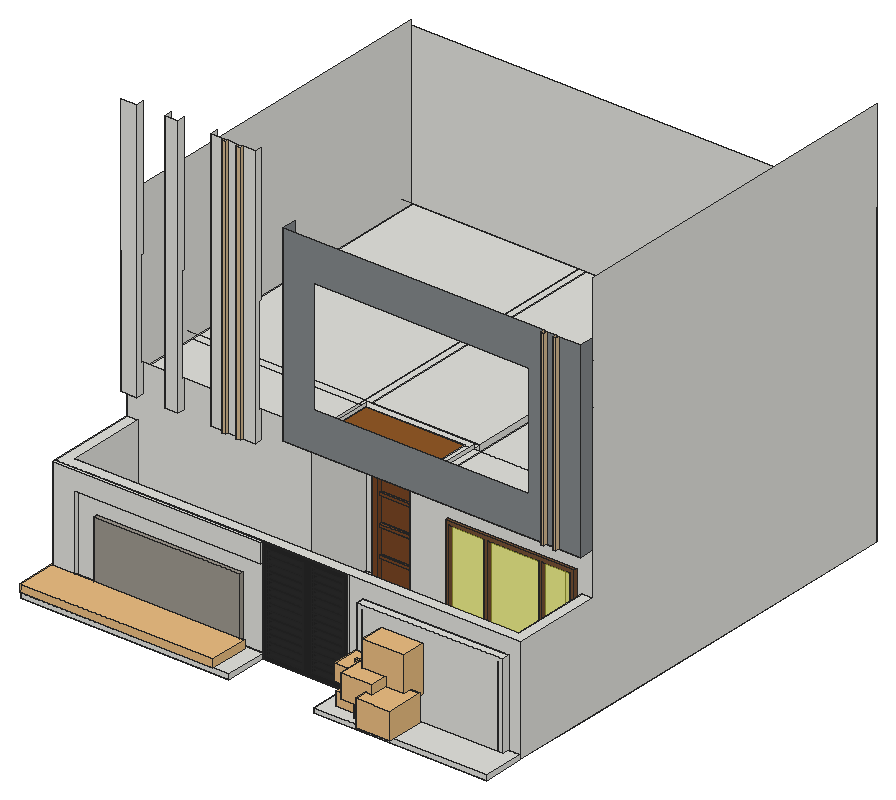
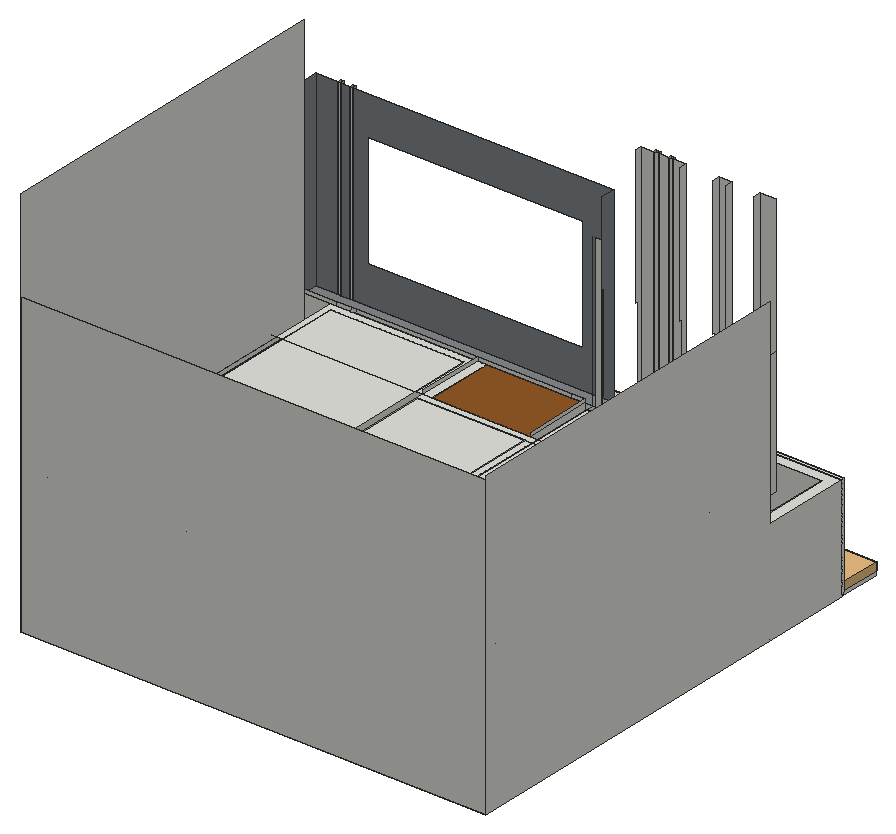
# SketchUp Ruby script. Lengths in inches.
U = 1.inch
M = Sketchup.active_model
def pt(a) = Geom::Point3d.new(a.map { |v| v * U })
def face(e, loops, mat)
  f = e.add_face(loops[0].map { |a| pt(a) })
  loops[1..].each { |l| e.add_face(l.map { |a| pt(a) }).erase! }
  f.material = f.back_material = mat if mat
  f
end
# faces: each face lists its corners as indices into pts; further lists are holes
def faces(e, pts, list, mat = nil) = list.each { |f| face(e, (f[0].is_a?(Array) ? f : [f]).map { |l| l.map { |i| pts[i] } }, mat) }
# xy, xz, yz: faces in a plane at the given z, y or x. An outline is a flat list of corners, or four numbers for a rectangle; further outlines are holes
def ring(l) = l.size == 4 ? [[l[0], l[1]], [l[2], l[1]], [l[2], l[3]], [l[0], l[3]]] : l.each_slice(2).to_a
def flat(e, list, mat, &to3) = list.each { |f| face(e, (f[0].is_a?(Array) ? f : [f]).map { |l| ring(l).map { |u, v| to3.(u, v) } }, mat) }
def xy(e, z, list, mat = nil) = flat(e, list, mat) { |x, y| [x, y, z] }
def xz(e, y, list, mat = nil) = flat(e, list, mat) { |x, z| [x, y, z] }
def yz(e, x, list, mat = nil) = flat(e, list, mat) { |y, z| [x, y, z] }
def lines(e, pts, list) = list.each { |a, b| e.add_line(pt(pts[a]), pt(pts[b])) }
# prism: a flat outline (further loops are holes) pulled along v
def prism(e, loops, v, mat = nil)
  f = face(e, loops, mat); d = Geom::Vector3d.new(v.map { |x| x * U })
  f.pushpull(f.normal.samedirection?(d) ? d.length : -d.length)
end
def box(e, o, s, mat = nil) = prism(e, [[o, [o[0] + s[0], o[1], o[2]], [o[0] + s[0], o[1] + s[1], o[2]], [o[0], o[1] + s[1], o[2]]]], [0, 0, s[2]], mat)
def at(x, y, z, deg = 0) = Geom::Transformation.translation(pt([x, y, z])) * Geom::Transformation.rotation(ORIGIN, Z_AXIS, deg.degrees)
def axes(o, x, y, z) = Geom::Transformation.new([*x, 0, *y, 0, *z, 0, *pt(o).to_a, 1])
def part(name) = M.definitions.add(name)
# library, detail: a bought-in or finely detailed component or shape, given as its bounding box
def library(name, o, s) = part(name).tap { |d| box(d.entities, o, s) }
def detail(e, o, s) = box(e.add_group.entities, o, s)
def put(e, d, t, mat = nil) = e.add_instance(d, t).tap { |i| i.material = mat if mat }
def group(e, t, mat = nil) = e.add_group.tap { |g| g.transformation = t; g.material = mat if mat }.entities
root = M.entities
M.materials.add("Material__1").color = [95, 70, 46]
M.materials.add("Material__2").color = [150, 168, 104]
M.materials.add("Material__3").color = [234, 233, 231]
M.materials.add("Material__4").color = [36, 36, 36]
M.materials.add("Material__5").color = [151, 172, 33]
M.materials.add("Material__6").color = [79, 108, 5]
M.materials.add("[0033_NavajoWhite]").color = [214, 186, 145]
M.materials.add("[0035_Tan]").color = [210, 180, 140]
M.materials.add("[0137_Black]").color = [40, 40, 40]
M.materials.add("[Blacktop Old 01]").color = [132, 136, 139]
M.materials.add("[Sandstone]").color = [118, 81, 52]
M.materials.add("[Stone Masonry Multi]").color = [158, 152, 142]
M.materials.add("[Translucent Glass Blue]").color = [254, 255, 58]
M.materials["[Translucent Glass Blue]"].alpha = 0.5
M.materials.add("[Wood Floor Parquet]").color = [145, 89, 39]
M.materials.add("[Wood Veneer 01]").color = [120, 70, 37]
M.materials.add("wire_1").color = [140, 184, 58]
M.materials.add("wire_2").color = [244, 244, 244]
M.materials.add("wire_4").color = [86, 225, 198]
M.materials.add("wire_5").color = [232, 232, 232]
c1 = library("Untitled.bahçe+çiçek+bitki+zemin+alanları",[0,-19.69,0],[135.94,19.69,5.51])
c2 = library("Group\#1",[-915.9375,-34.5,735.6],[41.04,40.85,6.81])
c3 = library("Group\#2",[-991.92,-34.05,729.49],[10.64,7.28,57.53])
c4 = library("Group\#3",[-1022.2,-71.69,736.68],[86.94,78.77,45.64])
c5 = library("Group\#4",[-877.77,-100.41,669.81],[37.9,37.9,42.75])
c6 = library("Group\#5",[-957.79,-83.08,701.98],[44.29,44.29,27.78])
c7 = library("Group\#6",[-1023.9,-65.47,669.625],[67.53,67.55,39.17])
c8 = library("Group\#7",[-997.48,-49.45,708.79],[29.81,29.81,30.61])
c9 = library("Group\#8",[-956738.95,-82059.81,669752.625],[42194.58,42232.57,49521.48])
c10 = library("Group\#9",[-917.52,-36.6875,711.84],[44.99,44.98,28.22])
c11 = library("Group\#10",[-916244.63,-35413.97,669800.48],[42442.38,42642.99,59706.29])
c12 = library("Group\#11",[-955.48,-54.29,730.4],[118.63,83.7,130.4])
c13 = library("Group\#12",[-899.97,-18.72,732.17],[8.78,8.27,28.64])
c14 = library("Group\#13",[-906.16,-138.28,686.8],[98.25,106.18,75.79])
c15 = library("Group\#14",[-978.71,-103.24,719.12],[90.2,76.4,68.29])
c16 = library("Group\#15",[-955.98,-81.17,725.57],[41.03,40.85,6.81])
c17 = library("Group\#16",[-996.8,-48.73,736.67],[28.51,28.38,4.73])
c18 = library("Group\#17",[-876.58,-99.29,706.19],[35.74,35.58,5.93])
c19 = library("Group\#18",[-912.1,-32.49,735.82],[33.14,36.63,9.55])
c20 = library("Group\#19",[-994.36,-46.95,735.88],[24.38,25.9,6.88])
c21 = part("PLANT-30")
p = [[0,0,0],[1,0,0],[1,1,0]]
lines(c21.entities,p,[[0,1],[1,2],[2,0]])
put(c21.entities,c2,at(895.63,-7.06,-669.82),"Material__1")
put(c21.entities,c3,at(895.63,-7.06,-669.82),"wire_1")
put(c21.entities,c4,at(895.63,-7.06,-669.82),"Material__2")
put(c21.entities,c5,at(895.63,-7.06,-669.82),"wire_2")
put(c21.entities,c6,at(895.63,-7.06,-669.82),"wire_2")
put(c21.entities,c7,at(895.63,-7.06,-669.82),"Material__3")
put(c21.entities,c8,at(895.63,-7.06,-669.82),"wire_2")
put(c21.entities,c9,axes([895.63,-7.06,-669.82],[0.001,0,0],[0,0.001,0],[0,0,0.001]),"Material__4")
put(c21.entities,c10,at(895.63,-7.06,-669.82),"wire_2")
put(c21.entities,c11,axes([895.63,-7.06,-669.82],[0.001,0,0],[0,0.001,0],[0,0,0.001]),"Material__4")
put(c21.entities,c12,at(895.63,-7.06,-669.82),"Material__5")
put(c21.entities,c13,at(895.63,-7.06,-669.82),"wire_4")
put(c21.entities,c14,at(895.63,-7.06,-669.82),"Material__6")
put(c21.entities,c15,at(895.63,-7.06,-669.82),"Material__4")
put(c21.entities,c16,at(895.63,-7.06,-669.82),"Material__1")
put(c21.entities,c17,at(895.63,-7.06,-669.82),"Material__1")
put(c21.entities,c18,at(895.63,-7.06,-669.82),"Material__1")
put(c21.entities,c19,at(895.63,-7.06,-669.82),"wire_5")
put(c21.entities,c20,at(895.63,-7.06,-669.82),"wire_5")
xy(root,-0.02,[[250.16,27.78,250.1,33.78,367.46,34.85,367.51,28.85]])
xy(root,0,[[0,0,18.1,31.8125],[18.1,0,168.7,34.8125],[237.67,0,377.5,33.8125],[0,31.8125,18.1,34.8125],[168.7,33.8125,238.07,34.8125],
  [0,34.8125,0,107.5,149.5625,107.5,149.5625,162.625,159.26,162.625,159.26,156.625,164.11,156.625,164.11,159.625,202.93,159.625,202.93,156.625,207.26,156.625,207.26,162.625,229.5625,162.625,229.5625,107.5,360,107.5,360,34.8125],[360,34.8125,377.5,107.5],[[0,107.5,0,394.8125,377.5,394.8125,377.5,107.5,229.5625,107.5,229.5625,162.625,149.5625,162.625,149.5625,107.5],[9,113.5,143.5625,385.8125],[242.6875,113.5,351,385.8125],[149.5625,168.625,236.6875,385.8125]],[9,113.5,143.5625,385.8125],[242.6875,113.5,351,385.8125],
  [159.26,156.625,164.11,159.625],[202.93,156.625,207.26,159.625],[159.26,159.625,207.26,162.625],[149.5625,168.625,236.6875,385.8125]])
xy(root,1,[[9,43.8125,368.5,43.8125,368.5,107.5,229.5625,107.5,229.5625,162.625,207.26,162.625,207.26,156.625,202.93,156.625,202.93,159.625,164.11,159.625,164.11,156.625,159.26,156.625,159.26,162.625,149.5625,162.625,149.5625,107.5,9,107.5]])
xy(root,3.88,[[0,0,168.7,0,168.7,34.8125,152.32,34.8125,152.32,31.8125,33.9375,31.8125,33.9375,34.8125,18.1,34.8125,18.1,31.8125,0,31.8125],[237.67,0,377.5,0,377.5,33.8125,363.57,33.8125,363.59,31.8125,254.03,30.8125,254,33.8125,237.67,33.8125],[254.03,30.8125,363.59,31.8125,363.57,33.8125,254,33.8125],[33.9375,31.8125,152.32,34.8125],[254,33.8125,363.5625,34.8125,363.57,33.8125]])
xy(root,3.95,[[172.65,33.8125,201.57,34.8125],[209.11,33.8125,234.125,34.8125],[172.65,34.8125,201.57,43.8125],[209.11,34.8125,234.125,43.8125]],"[0137_Black]")
xy(root,7.12,[[172.65,34.8125,201.57,43.8125],[209.11,34.8125,234.125,43.8125]],"[0137_Black]")
xy(root,9.21,[[172.65,34.8125,201.57,43.8125],[209.11,34.8125,234.125,43.8125]],"[0137_Black]")
xy(root,12.8,[[172.65,34.8125,201.57,43.8125],[209.11,34.8125,234.125,43.8125]],"[0137_Black]")
xy(root,14.9,[[172.65,34.8125,201.57,43.8125],[209.11,34.8125,234.125,43.8125]],"[0137_Black]")
xy(root,17.21,[[164.11,157.625,202.93,159.625]],"[Wood Veneer 01]")
xy(root,18.49,[[172.65,34.8125,201.57,43.8125],[209.11,34.8125,234.125,43.8125]],"[0137_Black]")
xy(root,19.52,[[164.11,157.625,202.93,159.625]],"[Wood Veneer 01]")
xy(root,20.59,[[172.65,34.8125,201.57,43.8125],[209.11,34.8125,234.125,43.8125]],"[0137_Black]")
xy(root,24.18,[[172.65,34.8125,201.57,43.8125],[209.11,34.8125,234.125,43.8125]],"[0137_Black]")
xy(root,24.5625,[[260.4,104.5,364.71,107.5]])
xy(root,26.28,[[172.65,34.8125,201.57,43.8125],[209.11,34.8125,234.125,43.8125]],"[0137_Black]")
xy(root,27.5625,[[263.4,104.5,291.4,107.5],[294.71,104.5,335.9,107.5],[338.84,104.5,361.71,107.5]],"[Sandstone]")
xy(root,29.87,[[172.65,34.8125,201.57,43.8125],[209.11,34.8125,234.125,43.8125]],"[0137_Black]")
xy(root,31.96,[[172.65,34.8125,201.57,43.8125],[209.11,34.8125,234.125,43.8125]],"[0137_Black]")
xy(root,35.55,[[172.65,34.8125,201.57,43.8125],[209.11,34.8125,234.125,43.8125]],"[0137_Black]")
xy(root,37.65,[[172.65,34.8125,201.57,43.8125],[209.11,34.8125,234.125,43.8125]],"[0137_Black]")
xy(root,40.15,[[164.11,157.625,202.93,159.625]],"[Wood Veneer 01]")
xy(root,41.24,[[172.65,34.8125,201.57,43.8125],[209.11,34.8125,234.125,43.8125]],"[0137_Black]")
xy(root,42.46,[[164.11,157.625,202.93,159.625]],"[Wood Veneer 01]")
xy(root,43.34,[[172.65,34.8125,201.57,43.8125],[209.11,34.8125,234.125,43.8125]],"[0137_Black]")
xy(root,46.93,[[172.65,34.8125,201.57,43.8125],[209.11,34.8125,234.125,43.8125]],"[0137_Black]")
xy(root,49.03,[[172.65,34.8125,201.57,43.8125],[209.11,34.8125,234.125,43.8125]],"[0137_Black]")
xy(root,52.62,[[172.65,34.8125,201.57,43.8125],[209.11,34.8125,234.125,43.8125]],"[0137_Black]")
xy(root,54.71,[[172.65,34.8125,201.57,43.8125],[209.11,34.8125,234.125,43.8125]],"[0137_Black]")
xy(root,57.0625,[[33.9375,31.8125,152.32,34.8125]],"[Stone Masonry Multi]")
xy(root,58.3,[[172.65,34.8125,201.57,43.8125],[209.11,34.8125,234.125,43.8125]],"[0137_Black]")
xy(root,60.4,[[172.65,34.8125,201.57,43.8125],[209.11,34.8125,234.125,43.8125]],"[0137_Black]")
xy(root,63.09,[[164.11,157.625,202.93,159.625]],"[Wood Veneer 01]")
xy(root,63.99,[[172.65,34.8125,201.57,43.8125],[209.11,34.8125,234.125,43.8125]],"[0137_Black]")
xy(root,65.4,[[164.11,157.625,202.93,159.625]],"[Wood Veneer 01]")
xy(root,66.09,[[172.65,34.8125,201.57,43.8125],[209.11,34.8125,234.125,43.8125]],"[0137_Black]")
xy(root,68.35,[[254.05,27.8125,254.03,30.8125,363.59,31.8125,363.62,28.8125],[254.03,30.8125,254,33.8125,363.5625,34.8125,363.59,31.8125]])
xy(root,69.68,[[172.65,34.8125,201.57,43.8125],[209.11,34.8125,234.125,43.8125]],"[0137_Black]")
xy(root,69.82,[[18.1,31.8125,168.7,34.8125]])
xy(root,71.78,[[172.65,34.8125,201.57,43.8125],[209.11,34.8125,234.125,43.8125]],"[0137_Black]")
xy(root,72.25,[[250.16,27.78,367.51,28.85,367.46,34.85,250.1,33.78]])
xy(root,75.37,[[172.65,34.8125,201.57,43.8125],[209.11,34.8125,234.125,43.8125]],"[0137_Black]")
xy(root,77.46,[[172.65,34.8125,201.57,43.8125],[209.11,34.8125,234.125,43.8125]],"[0137_Black]")
xy(root,80.14,[[164.11,156.625,202.93,159.625]],"[Wood Veneer 01]")
xy(root,81.05,[[172.65,33.8125,201.57,34.8125],[209.11,33.8125,234.125,34.8125],[172.65,34.8125,201.57,43.8125],[209.11,34.8125,234.125,43.8125]],"[0137_Black]")
xy(root,84,[[159.26,156.625,207.26,162.625]],"[Wood Veneer 01]")
xy(root,85,[[0,31.8125,168.7,34.8125],[0,34.8125,377.5,34.8125,377.5,107.5,368.5,107.5,368.5,43.8125,9,43.8125,9,107.5,0,107.5]])
xy(root,85,[[168.7,33.8125,238.07,34.8125]],"[0137_Black]")
xy(root,99.25,[[263.4,104.5,291.4,107.5],[294.71,104.5,335.9,107.5],[338.84,104.5,361.71,107.5]],"[Sandstone]")
xy(root,102.25,[[260.4,104.5,364.71,107.5]],"[Sandstone]")
xy(root,105.4375,[[0,101.5,12.9375,107.5],[35.3125,101.5,45.625,107.5],[72.45,101.5,108.79,107.5]])
xy(root,105.4375,[[82.86,99.5,86.5,101.5],[94.93,99.5,98.5625,101.5]],"[0033_NavajoWhite]")
xy(root,120,[[135.89,95.5,135.96,107.5],[229.5625,107.5,236.6875,162.625],[236.6875,107.5,236.6875,162.625,242.6875,162.625,242.6875,113.5,351,113.5,351,162.625,355.66,162.625,355.66,107.5],[9,113.5,143.5625,162.625],[242.6875,113.5,351,162.625],
  [9,162.625,143.5625,168.625],[143.5625,162.625,236.6875,168.625],[242.6875,162.625,351,385.8125],[9,168.625,143.5625,385.8125],[143.5625,168.625,149.5625,385.8125],
  [149.5625,168.625,236.6875,385.8125]])
xy(root,120,[[347.36,92.5,350.01,95.5],[357.24,92.5,359.89,95.5]],"[0033_NavajoWhite]")
xy(root,120,[[135.96,95.5,377.5,107.5]],"[Blacktop Old 01]")
xy(root,120,[[149.5625,107.5,229.5625,162.625]],"[Wood Floor Parquet]")
xz(root,0,[[0,0,168.7,3.88],[237.67,0,377.5,3.88]])
xz(root,31.8125,[[0,0,18.1,3.88],[0,3.88,18.1,3.88,18.1,69.82,168.7,69.82,168.7,85,0,85]])
xz(root,31.8125,[[33.9375,3.88,152.32,57.0625]],"[Stone Masonry Multi]")
xz(root,33.8125,[[237.67,0,238.07,3.88],[238.07,0,377.5,3.88]])
xz(root,33.8125,[[[168.7,0,237.67,0,237.67,3.88,238.07,3.88,238.07,85,168.7,85],[172.65,3.95,201.57,81.05],[209.11,3.95,234.125,81.05]]],"[0137_Black]")
xz(root,34.8125,[[0,0,0,85,168.7,85,168.7,69.82,18.1,69.82,18.1,0],[18.1,0,168.7,3.88],[[168.7,0,238.07,85],[172.65,3.95,201.57,81.05],[209.11,3.95,234.125,81.05]],[238.07,0,377.5,85],[18.1,3.88,33.9375,3.88,33.9375,57.0625,152.32,57.0625,152.32,3.88,168.7,3.88,168.7,69.82,18.1,69.82]])
xz(root,34.8125,[[172.65,7.12,201.57,9.21],[209.11,7.12,234.125,9.21],[172.65,12.8,201.57,14.9],[209.11,12.8,234.125,14.9],[172.65,18.49,201.57,20.59],
  [209.11,18.49,234.125,20.59],[172.65,24.18,201.57,26.28],[209.11,24.18,234.125,26.28],[172.65,29.87,201.57,31.96],[209.11,29.87,234.125,31.96],
  [172.65,35.55,201.57,37.65],[209.11,35.55,234.125,37.65],[172.65,41.24,201.57,43.34],[209.11,41.24,234.125,43.34],[172.65,46.93,201.57,49.03],
  [209.11,46.93,234.125,49.03],[172.65,52.62,201.57,54.71],[209.11,52.62,234.125,54.71],[172.65,58.3,201.57,60.4],[209.11,58.3,234.125,60.4],
  [172.65,63.99,201.57,66.09],[209.11,63.99,234.125,66.09],[172.65,69.68,201.57,71.78],[209.11,69.68,234.125,71.78],[172.65,75.37,201.57,77.46],
  [209.11,75.37,234.125,77.46]],"[0137_Black]")
xz(root,43.8125,[[[9,1,360,85],[172.65,71.78,201.57,75.37],[172.65,77.46,201.57,81.05],[172.65,66.09,201.57,69.68],[172.65,60.4,201.57,63.99],[172.65,54.71,201.57,58.3],[172.65,49.03,201.57,52.62],[172.65,43.34,201.57,46.93],[172.65,37.65,201.57,41.24],[172.65,31.96,201.57,35.55],[172.65,26.28,201.57,29.87],[172.65,20.59,201.57,24.18],[172.65,14.9,201.57,18.49],[172.65,9.21,201.57,12.8],[172.65,3.95,201.57,7.12],[209.11,9.21,234.125,12.8],[209.11,26.28,234.125,29.87],[209.11,14.9,234.125,18.49],[209.11,77.46,234.125,81.05],[209.11,71.78,234.125,75.37],[209.11,66.09,234.125,69.68],[209.11,60.4,234.125,63.99],[209.11,54.71,234.125,58.3],[209.11,49.03,234.125,52.62],[209.11,43.34,234.125,46.93],[209.11,37.65,234.125,41.24],[209.11,20.59,234.125,24.18],[209.11,31.96,234.125,35.55],[209.11,3.95,234.125,7.12]],[360,1,368.5,85]])
xz(root,92.5,[[347.36,120,350.01,274.3125],[357.24,120,359.89,274.3125]],"[0033_NavajoWhite]")
xz(root,95.5,[[135.89,120,135.96,243],[347.36,120,350.01,274.3125],[357.24,120,359.89,274.3125]])
xz(root,95.5,[[[135.96,120,347.36,120,347.36,274.3125,135.89,274.3125,135.89,243,135.96,243],[160.6875,150.99,335.27,243]],[350.01,120,357.24,274.3125],[359.89,120,377.5,274.3125]],"[Blacktop Old 01]")
xz(root,99.5,[[82.86,105.4375,86.5,318],[94.93,105.4375,98.5625,318]],"[0033_NavajoWhite]")
xz(root,101.5,[[0,105.4375,12.9375,318],[35.3125,105.4375,45.625,318],[72.45,105.4375,82.86,318],[82.86,105.4375,86.5,318],[86.5,105.4375,94.93,318],
  [94.93,105.4375,98.5625,318],[98.5625,105.4375,108.79,318]])
xz(root,104.5,[[[260.4,24.5625,364.71,102.25],[294.71,27.5625,335.9,99.25],[263.4,27.5625,291.4,99.25],[338.84,27.5625,361.71,99.25]]],"[Sandstone]")
xz(root,107.5,[[229.5625,0,360,1],[9,1,149.5625,1,149.5625,120,135.89,120,135.89,128.33,108.79,128.33,108.79,105.4375,72.45,105.4375,72.45,128.33,45.625,128.33,45.625,105.4375,35.3125,105.4375,35.3125,128.33,12.9375,128.33,12.9375,105.4375,0,105.4375,0,85,9,85],[[229.5625,1,368.5,1,368.5,85,377.5,85,377.5,120,229.5625,120],[260.4,24.5625,364.71,102.25]],[[260.4,24.5625,364.71,102.25],[294.71,27.5625,335.9,99.25],[263.4,27.5625,291.4,99.25],[338.84,27.5625,361.71,99.25]],[0,105.4375,12.9375,128.33],
  [35.3125,105.4375,45.625,128.33],[72.45,105.4375,108.79,128.33],[135.89,120,135.96,243],[135.96,120,140.5625,243],[149.5625,120,151.6875,123],
  [151.6875,120,160.6875,123],[160.6875,120,236.6875,123],[236.6875,120,335.27,123],[335.27,120,339.25,123],[339.25,120,351,123],
  [351,120,377.5,123]])
xz(root,107.5,[[263.4,27.5625,291.4,99.25],[294.71,27.5625,335.9,99.25],[338.84,27.5625,361.71,99.25]],"[Translucent Glass Blue]")
xz(root,113.5,[[9,0,143.5625,120],[242.6875,0,351,120]])
xz(root,156.625,[[159.26,0,164.11,1],[202.93,0,207.26,1]])
xz(root,156.625,[[159.26,1,164.11,1,164.11,80.14,202.93,80.14,202.93,1,207.26,1,207.26,84,159.26,84]],"[Wood Veneer 01]")
xz(root,157.625,[[164.11,17.21,202.93,19.52],[164.11,40.15,202.93,42.46],[164.11,63.09,202.93,65.4]],"[Wood Veneer 01]")
xz(root,159.625,[[164.11,0,202.93,1],[164.11,17.21,202.93,19.52],[164.11,40.15,202.93,42.46],[164.11,63.09,202.93,65.4]])
xz(root,159.625,[[164.11,1,202.93,17.21],[164.11,19.52,202.93,40.15],[164.11,42.46,202.93,63.09],[164.11,65.4,202.93,80.14]],"[Wood Veneer 01]")
xz(root,162.625,[[149.5625,0,159.26,1],[159.26,0,207.26,84],[207.26,0,229.5625,1],[149.5625,1,159.26,1,159.26,84,207.26,84,207.26,1,229.5625,1,229.5625,120,149.5625,120]])
xz(root,168.625,[[149.5625,0,236.6875,120]])
xz(root,385.8125,[[9,0,143.5625,120],[149.5625,0,236.6875,120],[242.6875,0,351,120]])
xz(root,394.8125,[[0,0,377.5,243]])
yz(root,0,[[0,0,31.8125,3.88],[31.8125,0,34.8125,85],[34.8125,0,34.8125,85,107.5,85,107.5,246,394.8125,246,394.8125,0],[101.5,105.4375,107.5,207.1]])
yz(root,9,[[113.5,0,385.8125,120],[43.8125,1,107.5,85]])
yz(root,12.9375,[[101.5,105.4375,107.5,105.4375,107.5,128.33,105.5,128.33,105.5,207.1,107.5,207.1,107.5,318,101.5,318]])
yz(root,18.1,[[31.8125,0,34.8125,3.88],[31.8125,3.88,34.8125,69.82]])
yz(root,33.9375,[[31.8125,3.88,34.8125,57.0625]],"[Stone Masonry Multi]")
yz(root,35.3125,[[101.5,105.4375,101.5,318,107.5,318,107.5,207.1,105.5,207.1,105.5,128.33,107.5,128.33,107.5,105.4375]])
yz(root,45.625,[[101.5,105.4375,107.5,105.4375,107.5,128.33,105.5,128.33,105.5,207.1,107.5,207.1,107.5,318,101.5,318]])
yz(root,72.45,[[101.5,105.4375,101.5,318,107.5,318,107.5,207.1,105.5,207.1,105.5,128.33,107.5,128.33,107.5,105.4375]])
yz(root,82.86,[[99.5,105.4375,101.5,318]],"[0033_NavajoWhite]")
yz(root,86.5,[[99.5,105.4375,101.5,318]],"[0033_NavajoWhite]")
yz(root,94.93,[[99.5,105.4375,101.5,318]],"[0033_NavajoWhite]")
yz(root,98.5625,[[99.5,105.4375,101.5,318]],"[0033_NavajoWhite]")
yz(root,108.79,[[101.5,105.4375,107.5,105.4375,107.5,128.33,105.5,128.33,105.5,207.1,107.5,207.1,107.5,318,101.5,318]])
yz(root,135.89,[[95.5,120,95.5,274.3125,107.5,274.3125,107.5,207.1,105.5,207.1,105.5,128.33,107.5,128.33,107.5,120]],"[Blacktop Old 01]")
yz(root,143.5625,[[113.5,0,385.8125,120]])
yz(root,149.5625,[[107.5,0,162.625,1],[168.625,0,385.8125,120],[107.5,1,162.625,120],[107.5,120,162.625,123]])
yz(root,152.32,[[31.8125,3.88,34.8125,57.0625]],"[Stone Masonry Multi]")
yz(root,159.26,[[156.625,0,159.625,1],[159.625,0,162.625,1]])
yz(root,159.26,[[156.625,1,162.625,84]],"[Wood Veneer 01]")
yz(root,164.11,[[156.625,0,159.625,1],[157.625,17.21,159.625,19.52],[157.625,40.15,159.625,42.46],[157.625,63.09,159.625,65.4]])
yz(root,164.11,[[156.625,1,159.625,1,159.625,17.21,157.625,17.21,157.625,19.52,159.625,19.52,159.625,40.15,157.625,40.15,157.625,42.46,159.625,42.46,159.625,63.09,157.625,63.09,157.625,65.4,159.625,65.4,159.625,80.14,156.625,80.14]],"[Wood Veneer 01]")
yz(root,168.7,[[0,0,33.8125,3.88],[33.8125,0,34.8125,3.88],[33.8125,3.88,34.8125,69.82],[31.8125,69.82,33.8125,85],[33.8125,69.82,34.8125,85]])
yz(root,172.65,[[33.8125,3.95,34.8125,7.12],[34.8125,3.95,43.8125,7.12],[33.8125,7.12,34.8125,9.21],[33.8125,9.21,34.8125,12.8],[34.8125,9.21,43.8125,12.8],
  [33.8125,12.8,34.8125,14.9],[33.8125,14.9,34.8125,18.49],[34.8125,14.9,43.8125,18.49],[33.8125,18.49,34.8125,20.59],[33.8125,20.59,34.8125,24.18],
  [34.8125,20.59,43.8125,24.18],[33.8125,24.18,34.8125,26.28],[33.8125,26.28,34.8125,29.87],[34.8125,26.28,43.8125,29.87],[33.8125,29.87,34.8125,31.96],
  [33.8125,31.96,34.8125,35.55],[34.8125,31.96,43.8125,35.55],[33.8125,35.55,34.8125,37.65],[33.8125,37.65,34.8125,41.24],[34.8125,37.65,43.8125,41.24],
  [33.8125,41.24,34.8125,43.34],[33.8125,43.34,34.8125,46.93],[34.8125,43.34,43.8125,46.93],[33.8125,46.93,34.8125,49.03],[33.8125,49.03,34.8125,52.62],
  [34.8125,49.03,43.8125,52.62],[33.8125,52.62,34.8125,54.71],[33.8125,54.71,34.8125,58.3],[34.8125,54.71,43.8125,58.3],[33.8125,58.3,34.8125,60.4],
  [33.8125,60.4,34.8125,63.99],[34.8125,60.4,43.8125,63.99],[33.8125,63.99,34.8125,66.09],[33.8125,66.09,34.8125,69.68],[34.8125,66.09,43.8125,69.68],
  [33.8125,69.68,34.8125,71.78],[33.8125,71.78,34.8125,75.37],[34.8125,71.78,43.8125,75.37],[33.8125,75.37,34.8125,77.46],[33.8125,77.46,34.8125,81.05],
  [34.8125,77.46,43.8125,81.05]],"[0137_Black]")
yz(root,201.57,[[33.8125,3.95,34.8125,7.12],[34.8125,3.95,43.8125,7.12],[33.8125,7.12,34.8125,9.21],[33.8125,9.21,34.8125,12.8],[34.8125,9.21,43.8125,12.8],
  [33.8125,12.8,34.8125,14.9],[33.8125,14.9,34.8125,18.49],[34.8125,14.9,43.8125,18.49],[33.8125,18.49,34.8125,20.59],[33.8125,20.59,34.8125,24.18],
  [34.8125,20.59,43.8125,24.18],[33.8125,24.18,34.8125,26.28],[33.8125,26.28,34.8125,29.87],[34.8125,26.28,43.8125,29.87],[33.8125,29.87,34.8125,31.96],
  [33.8125,31.96,34.8125,35.55],[34.8125,31.96,43.8125,35.55],[33.8125,35.55,34.8125,37.65],[33.8125,37.65,34.8125,41.24],[34.8125,37.65,43.8125,41.24],
  [33.8125,41.24,34.8125,43.34],[33.8125,43.34,34.8125,46.93],[34.8125,43.34,43.8125,46.93],[33.8125,46.93,34.8125,49.03],[33.8125,49.03,34.8125,52.62],
  [34.8125,49.03,43.8125,52.62],[33.8125,52.62,34.8125,54.71],[33.8125,54.71,34.8125,58.3],[34.8125,54.71,43.8125,58.3],[33.8125,58.3,34.8125,60.4],
  [33.8125,60.4,34.8125,63.99],[34.8125,60.4,43.8125,63.99],[33.8125,63.99,34.8125,66.09],[33.8125,66.09,34.8125,69.68],[34.8125,66.09,43.8125,69.68],
  [33.8125,69.68,34.8125,71.78],[33.8125,71.78,34.8125,75.37],[34.8125,71.78,43.8125,75.37],[33.8125,75.37,34.8125,77.46],[33.8125,77.46,34.8125,81.05],
  [34.8125,77.46,43.8125,81.05]],"[0137_Black]")
yz(root,202.93,[[156.625,0,159.625,1],[157.625,17.21,159.625,19.52],[157.625,40.15,159.625,42.46],[157.625,63.09,159.625,65.4]])
yz(root,202.93,[[156.625,1,156.625,80.14,159.625,80.14,159.625,65.4,157.625,65.4,157.625,63.09,159.625,63.09,159.625,42.46,157.625,42.46,157.625,40.15,159.625,40.15,159.625,19.52,157.625,19.52,157.625,17.21,159.625,17.21,159.625,1]],"[Wood Veneer 01]")
yz(root,207.26,[[156.625,0,159.625,1],[159.625,0,162.625,1]])
yz(root,207.26,[[156.625,1,162.625,84]],"[Wood Veneer 01]")
yz(root,209.11,[[33.8125,3.95,34.8125,7.12],[34.8125,3.95,43.8125,7.12],[33.8125,7.12,34.8125,9.21],[33.8125,9.21,34.8125,12.8],[34.8125,9.21,43.8125,12.8],
  [33.8125,12.8,34.8125,14.9],[33.8125,14.9,34.8125,18.49],[34.8125,14.9,43.8125,18.49],[33.8125,18.49,34.8125,20.59],[33.8125,20.59,34.8125,24.18],
  [34.8125,20.59,43.8125,24.18],[33.8125,24.18,34.8125,26.28],[33.8125,26.28,34.8125,29.87],[34.8125,26.28,43.8125,29.87],[33.8125,29.87,34.8125,31.96],
  [33.8125,31.96,34.8125,35.55],[34.8125,31.96,43.8125,35.55],[33.8125,35.55,34.8125,37.65],[33.8125,37.65,34.8125,41.24],[34.8125,37.65,43.8125,41.24],
  [33.8125,41.24,34.8125,43.34],[33.8125,43.34,34.8125,46.93],[34.8125,43.34,43.8125,46.93],[33.8125,46.93,34.8125,49.03],[33.8125,49.03,34.8125,52.62],
  [34.8125,49.03,43.8125,52.62],[33.8125,52.62,34.8125,54.71],[33.8125,54.71,34.8125,58.3],[34.8125,54.71,43.8125,58.3],[33.8125,58.3,34.8125,60.4],
  [33.8125,60.4,34.8125,63.99],[34.8125,60.4,43.8125,63.99],[33.8125,63.99,34.8125,66.09],[33.8125,66.09,34.8125,69.68],[34.8125,66.09,43.8125,69.68],
  [33.8125,69.68,34.8125,71.78],[33.8125,71.78,34.8125,75.37],[34.8125,71.78,43.8125,75.37],[33.8125,75.37,34.8125,77.46],[33.8125,77.46,34.8125,81.05],
  [34.8125,77.46,43.8125,81.05]],"[0137_Black]")
yz(root,229.5625,[[107.5,0,162.625,1],[107.5,1,162.625,120]])
yz(root,234.125,[[33.8125,3.95,34.8125,7.12],[34.8125,3.95,43.8125,7.12],[33.8125,7.12,34.8125,9.21],[33.8125,9.21,34.8125,12.8],[34.8125,9.21,43.8125,12.8],
  [33.8125,12.8,34.8125,14.9],[33.8125,14.9,34.8125,18.49],[34.8125,14.9,43.8125,18.49],[33.8125,18.49,34.8125,20.59],[33.8125,20.59,34.8125,24.18],
  [34.8125,20.59,43.8125,24.18],[33.8125,24.18,34.8125,26.28],[33.8125,26.28,34.8125,29.87],[34.8125,26.28,43.8125,29.87],[33.8125,29.87,34.8125,31.96],
  [33.8125,31.96,34.8125,35.55],[34.8125,31.96,43.8125,35.55],[33.8125,35.55,34.8125,37.65],[33.8125,37.65,34.8125,41.24],[34.8125,37.65,43.8125,41.24],
  [33.8125,41.24,34.8125,43.34],[33.8125,43.34,34.8125,46.93],[34.8125,43.34,43.8125,46.93],[33.8125,46.93,34.8125,49.03],[33.8125,49.03,34.8125,52.62],
  [34.8125,49.03,43.8125,52.62],[33.8125,52.62,34.8125,54.71],[33.8125,54.71,34.8125,58.3],[34.8125,54.71,43.8125,58.3],[33.8125,58.3,34.8125,60.4],
  [33.8125,60.4,34.8125,63.99],[34.8125,60.4,43.8125,63.99],[33.8125,63.99,34.8125,66.09],[33.8125,66.09,34.8125,69.68],[34.8125,66.09,43.8125,69.68],
  [33.8125,69.68,34.8125,71.78],[33.8125,71.78,34.8125,75.37],[34.8125,71.78,43.8125,75.37],[33.8125,75.37,34.8125,77.46],[33.8125,77.46,34.8125,81.05],
  [34.8125,77.46,43.8125,81.05]],"[0137_Black]")
yz(root,236.6875,[[168.625,0,385.8125,120],[107.5,120,162.625,123]])
yz(root,237.67,[[0,0,33.8125,3.88]])
yz(root,238.07,[[33.8125,0,34.8125,85]])
yz(root,242.6875,[[113.5,0,385.8125,120]])
yz(root,260.4,[[104.5,24.5625,107.5,102.25]],"[Sandstone]")
yz(root,263.4,[[104.5,27.5625,107.5,99.25]],"[Sandstone]")
yz(root,291.4,[[104.5,27.5625,107.5,99.25]],"[Sandstone]")
yz(root,294.71,[[104.5,27.5625,107.5,99.25]],"[Sandstone]")
yz(root,335.9,[[104.5,27.5625,107.5,99.25]],"[Sandstone]")
yz(root,338.84,[[104.5,27.5625,107.5,99.25]],"[Sandstone]")
yz(root,347.36,[[92.5,120,95.5,274.3125]],"[0035_Tan]")
yz(root,350.01,[[92.5,120,95.5,274.3125]],"[0033_NavajoWhite]")
yz(root,351,[[113.5,0,385.8125,120]])
yz(root,357.24,[[92.5,120,95.5,274.3125]],"[0033_NavajoWhite]")
yz(root,359.89,[[92.5,120,95.5,274.3125]],"[0033_NavajoWhite]")
yz(root,361.71,[[104.5,27.5625,107.5,99.25]],"[Sandstone]")
yz(root,364.71,[[104.5,24.5625,107.5,102.25]],"[Sandstone]")
yz(root,368.5,[[43.8125,1,107.5,85]])
yz(root,377.5,[[0,0,33.8125,3.88],[34.8125,0,394.8125,0,394.8125,318,107.5,318,107.5,85,34.8125,85]])
yz(root,377.5,[[95.5,120,107.5,274.3125]],"[Blacktop Old 01]")
p = [[250.1,33.78,72.25],[250.1,33.78,-0.02],[250.16,27.78,-0.02],[250.16,27.78,72.25],[367.51,28.85,72.25],[367.51,28.85,-0.02],
  [367.46,34.85,-0.02],[367.46,34.85,72.25],[254,33.8125,68.35],[254,33.8125,3.88],[363.5625,34.8125,3.88],[363.5625,34.8125,68.35],
  [254.05,27.8125,3.88],[254.03,30.8125,3.88],[254.03,30.8125,68.35],[254.05,27.8125,68.35],[363.62,28.8125,68.35],[363.59,31.8125,68.35],
  [363.59,31.8125,3.88],[363.62,28.8125,3.88],[363.57,33.8125,3.88],[355.66,162.625,120],[360,162.625,120],[355.66,394.8125,120],
  [242.6875,385.8125,120],[242.6875,394.8125,120],[9,168.625,120],[0,168.625,120],[9,385.8125,120],[0,385.8125,120],
  [143.5625,113.5,120],[143.5625,107.5,120],[9,113.5,120],[9,107.5,120],[143.5625,107.5,243],[0,107.5,1],
  [9,107.5,1]]
faces(root,p,[[0,1,2,3],[4,3,2,5],[6,7,4,5],[[0,7,6,1],[8,9,10,11]],[12,13,14,15],[16,17,18,19],[14,13,18,17],[9,8,14,13],
  [11,10,20,18,17]])
lines(root,p,[[21,22],[21,23],[24,25],[26,27],[28,29],[30,31],[32,33],[34,31],[35,36]])
put(root,c1,axes([-0.49,31.87,3.88],[1.15,0,0],[0,1.61912,0],[0,0,1.15]))
put(root,c21,axes([286.93,25.5,7.64],[0.2814,0,0],[0,0.2814,0],[0,0,0.2814]))
